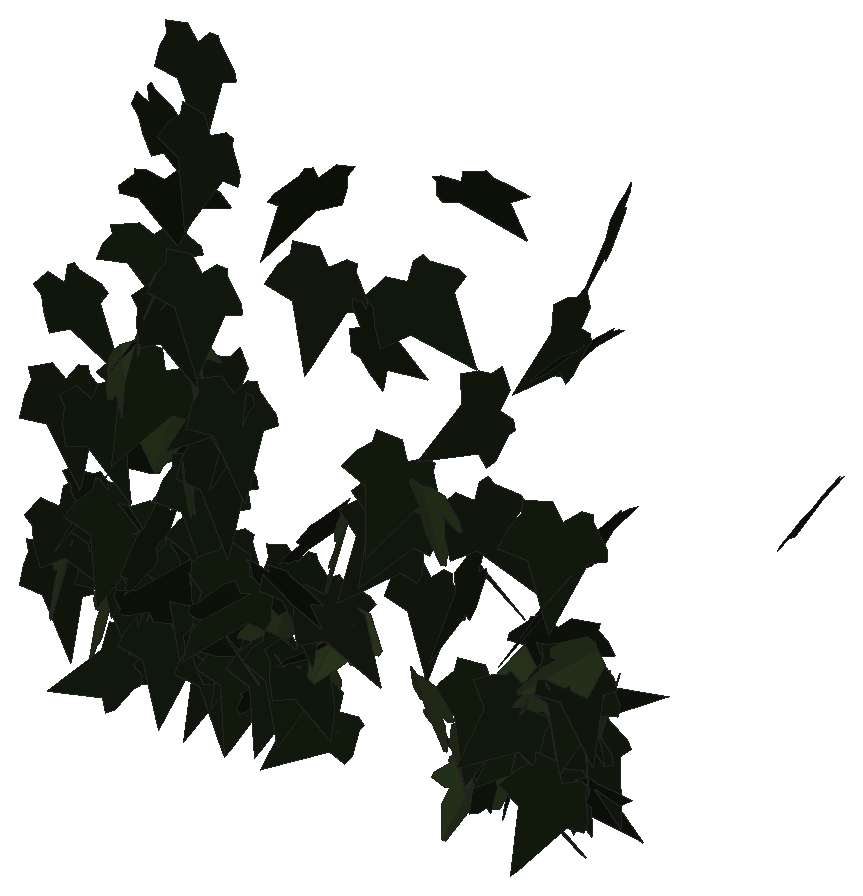
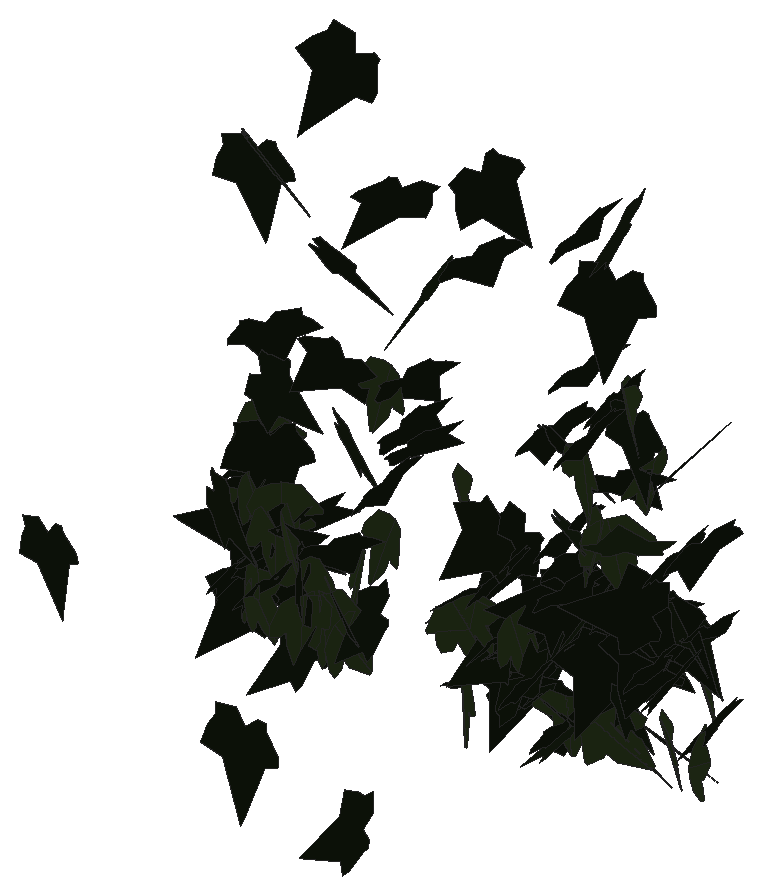
# SketchUp Ruby script. Lengths in inches.
U = 1.inch
M = Sketchup.active_model
def pt(a) = Geom::Point3d.new(a.map { |v| v * U })
def face(e, loops, mat)
  f = e.add_face(loops[0].map { |a| pt(a) })
  loops[1..].each { |l| e.add_face(l.map { |a| pt(a) }).erase! }
  f.material = f.back_material = mat if mat
  f
end
# faces: each face lists its corners as indices into pts; further lists are holes
def faces(e, pts, list, mat = nil) = list.each { |f| face(e, (f[0].is_a?(Array) ? f : [f]).map { |l| l.map { |i| pts[i] } }, mat) }
# xy, xz, yz: faces in a plane at the given z, y or x. An outline is a flat list of corners, or four numbers for a rectangle; further outlines are holes
def ring(l) = l.size == 4 ? [[l[0], l[1]], [l[2], l[1]], [l[2], l[3]], [l[0], l[3]]] : l.each_slice(2).to_a
def flat(e, list, mat, &to3) = list.each { |f| face(e, (f[0].is_a?(Array) ? f : [f]).map { |l| ring(l).map { |u, v| to3.(u, v) } }, mat) }
def xy(e, z, list, mat = nil) = flat(e, list, mat) { |x, y| [x, y, z] }
def xz(e, y, list, mat = nil) = flat(e, list, mat) { |x, z| [x, y, z] }
def yz(e, x, list, mat = nil) = flat(e, list, mat) { |y, z| [x, y, z] }
def lines(e, pts, list) = list.each { |a, b| e.add_line(pt(pts[a]), pt(pts[b])) }
# prism: a flat outline (further loops are holes) pulled along v
def prism(e, loops, v, mat = nil)
  f = face(e, loops, mat); d = Geom::Vector3d.new(v.map { |x| x * U })
  f.pushpull(f.normal.samedirection?(d) ? d.length : -d.length)
end
def box(e, o, s, mat = nil) = prism(e, [[o, [o[0] + s[0], o[1], o[2]], [o[0] + s[0], o[1] + s[1], o[2]], [o[0], o[1] + s[1], o[2]]]], [0, 0, s[2]], mat)
def at(x, y, z, deg = 0) = Geom::Transformation.translation(pt([x, y, z])) * Geom::Transformation.rotation(ORIGIN, Z_AXIS, deg.degrees)
def axes(o, x, y, z) = Geom::Transformation.new([*x, 0, *y, 0, *z, 0, *pt(o).to_a, 1])
def part(name) = M.definitions.add(name)
# library, detail: a bought-in or finely detailed component or shape, given as its bounding box
def library(name, o, s) = part(name).tap { |d| box(d.entities, o, s) }
def detail(e, o, s) = box(e.add_group.entities, o, s)
def put(e, d, t, mat = nil) = e.add_instance(d, t).tap { |i| i.material = mat if mat }
def group(e, t, mat = nil) = e.add_group.tap { |g| g.transformation = t; g.material = mat if mat }.entities
root = M.entities
M.materials.add("efeu1").color = [18, 25, 13]
M.materials.add("efeu2").color = [43, 57, 29]
c1 = part("ivyleaf_9")
p = [[1.54,2.16,1.25],[1.36,2.04,1.19],[-0.21,0.99,0.68],[-0.71,1.11,0.82],[-0.85,0.86,0.67],[-0.8,0.17,0.21],
  [-0.9,-0.01,0.1],[-0.67,-0.16,-0.02],[-0.08,-0.08,-0.05],[-0.03,-0.6,-0.4],[0.65,-0.88,-0.66],[0.83,-0.6,-0.49],
  [1.29,-0.42,-0.43],[1.8125,-0.07,-0.26],[1.21,0.44,0.15]]
faces(c1.entities,p,[[0,1,2,3,4,5,6,7,8,9,10,11,12,13,14]],"efeu1")
c2 = part("ivyleaf_10")
p = [[0,0.5,-0.03],[-0.0625,2.02,-0.43],[-0.19,2.01,-0.46],[-0.54,1.05,-0.29],[-0.52,0.625,-0.18],[-0.83,0.76,-0.28],
  [-1.16,0.64,-0.33],[-1.15,0.33,-0.24],[-0.77,-0.39,0.02],[-0.3,-0.51,0.16],[0.04,-0.48,0.23],[-0.02,2.01,-0.4375],
  [-0.06,2.01,-0.43],[0.04,-0.49,0.23],[0.67,-0.49,0.14],[1.38,0.36,-0.2],[1.375,0.51,-0.24],[0.81,0.65,-0.19],
  [0.62,0.59,-0.15],[0.6,1.09,-0.28],[0.5,1.23,-0.31]]
faces(c2.entities,p,[[0,1,2,3,4,5,6,7,8,9,10],[11,12,0,13,14,15,16,17,18,19,20]],"efeu2")
put(root,c1,axes([610.64,121.71,306.62],[1.08551,0.69081,0.17384],[-0.15041,-0.08744,1.28666],[0.69629,-1.09586,0.00692]))
put(root,c1,axes([614.42,122.42,308.86],[-1.10207,-0.62143,0.03852],[-0.02912,-0.02679,-1.26517],[0.62194,-1.10242,0.00903]))
put(root,c1,axes([618.05,122.52,322.72],[-0.41408,-1.25309,-0.00492],[0.02508,-0.00311,-1.3195],[1.25285,-0.4141,0.02479]))
put(root,c1,axes([610.88,121.58,309.32],[-0.86146,0.89959,0.31349],[-0.24442,0.19979,-1.24499],[-0.92076,-0.89469,0.03719]))
put(root,c1,axes([617.8,122.21,326.47],[-0.25735,0.84043,-0.97979],[0.18728,-0.9642,-0.87624],[-1.2772,-0.31073,0.06893]))
put(root,c1,axes([613.96,122.34,316.17],[0.01708,-1.28705,-0.21282],[0.02089,0.21308,-1.28695],[1.30436,0.01344,0.0234]))
put(root,c1,axes([621.48,122.69,315.9],[-0.56375,-1.14112,0.16814],[-0.04683,-0.16435,-1.27241],[1.15249,-0.56486,0.03055]))
put(root,c1,axes([621.02,122.91,312.99],[-0.6656,-0.96256,0.5463],[-0.13452,-0.5624,-1.15482],[1.09858,-0.65206,0.18958]))
put(root,c1,axes([626.11,122.16,319.94],[-1.26166,0.2257,0.22147],[-0.2124,0.07001,-1.28131],[-0.23426,-1.27904,-0.03105]))
put(root,c2,axes([623.17,121.78,307.72],[-1.10794,0.56302,-0.13169],[0.1236,-0.04743,-1.24271],[-0.56485,-1.11473,-0.01363]))
put(root,c1,axes([628.68,122.52,305.29],[-1.05697,-0.60589,-0.18367],[0.17173,0.06967,-1.21806],[0.60938,-1.07055,0.02468]))
put(root,c1,axes([612.33,122.9,326],[-0.13885,-1.22781,0.42385],[-0.04229,-0.42177,-1.23562],[1.29822,-0.14506,0.00508]))
put(root,c2,axes([606.21,122.37,307.05],[0.79546,-0.92167,0.22736],[0.14224,-0.17755,-1.21744],[0.93858,0.80804,-0.00818]))
put(root,c2,axes([629.6,122.72,310.77],[0.07849,0.50649,-1.15391],[-0.8251,-0.85322,-0.43063],[-0.9525,0.78083,0.27794]))
put(root,c1,axes([608.72,122.79,309.53],[-0.62675,-1.11366,-0.00561],[0.1299,-0.06671,-1.26955],[1.10607,-0.62321,0.14592]))
put(root,c1,axes([609.25,122.22,303.62],[-1.09457,0.48971,0.33079],[-0.38392,-0.05992,-1.18167],[-0.44927,-1.14189,0.20387]))
put(root,c1,axes([606.38,121.96,309.07],[0.53454,-1.03447,-0.68023],[-0.04926,0.72256,-1.13756],[1.23709,0.47576,0.24863]))
put(root,c1,axes([626.62,123.11,307.45],[-0.57289,-0.82169,0.75071],[-0.32175,-0.68601,-0.9964],[1.06546,-0.64897,0.10276]))
put(root,c1,axes([622.4375,121.84,323.98],[0.13632,-0.81519,-1.05838],[0.1734,1.06567,-0.79847],[1.32462,-0.05562,0.21344]))
put(root,c1,axes([616.21,121.72,309.96],[1.23253,0.18978,-0.27365],[-0.27289,-0.02575,-1.24695],[-0.19087,1.26228,0.0157]))
put(root,c1,axes([607.3,121.91,309.33],[-0.67909,1.04755,-0.01213],[0.00582,-0.01068,-1.24841],[-1.0476,-0.67911,0.00092]))
put(root,c1,axes([613.58,121.23,307.36],[0.30178,0.83143,-1.063],[0.10534,1.07142,0.86792],[1.34542,-0.27038,0.17048]))
put(root,c1,axes([625.12,121.62,329.21],[1.19782,0.60261,-0.08137],[-0.06909,-0.04373,-1.34084],[-0.60414,1.19978,-0.008]))
put(root,c1,axes([628.69,122.7,315.92],[-0.59992,-1.12921,-0.35348],[0.12369,0.3343,-1.27785],[1.17676,-0.61082,-0.0459]))
put(root,c2,axes([624.63,121.76,305.61],[-0.75004,0.83417,0.54696],[-0.40946,0.36656,-1.12051],[-0.90959,-0.85286,0.05339]))
put(root,c1,axes([628.76,122.77,313.43],[-0.79843,0.57207,-0.85057],[0.41945,-0.80142,-0.93275],[-0.93531,-0.84776,0.3078]))
put(root,c2,axes([608.98,122.27,315.89],[-0.0518,1.24886,-0.16149],[0.00177,-0.16155,-1.24993],[-1.25926,-0.0516,0.00489]))
put(root,c2,axes([622.96,122.24,315.18],[-1.21093,0.34721,-0.14431],[0.10606,-0.15147,-1.25441],[-0.36074,-1.21006,0.11562]))
put(root,c2,axes([610.1,122.39,318.86],[0.61528,-1.10104,-0.14151],[-0.05967,0.12876,-1.26125],[1.10849,0.61807,0.01065]))
put(root,c1,axes([610.26,122.25,326.84],[0.97872,-0.90264,-0.37513],[-0.27172,0.2587,-1.3314],[0.93897,1.01572,0.00573]))
put(root,c1,axes([621.17,123.27,313.94],[-0.43563,-1.10953,0.50024],[-0.19344,-0.46145,-1.19194],[1.20162,-0.47653,-0.01053]))
put(root,c1,axes([610.03,123.12,315.4375],[-0.94207,-0.86611,-0.0184],[0.10671,-0.08904,-1.27227],[0.8597,-0.93804,0.13776]))
put(root,c1,axes([611.83,123.1,320.05],[-0.12253,-1.29694,0.07763],[0.10807,-0.08788,-1.29757],[1.29475,-0.1154,0.11566]))
put(root,c1,axes([615.54,123.15,305.48],[-0.37744,-1.16583,0.13824],[-0.05775,-0.1266,-1.2253],[1.17258,-0.38151,-0.01585]))
put(root,c1,axes([605.84,122.84,313.69],[0.06407,-1.26811,-0.30251],[-0.05005,0.30026,-1.26928],[1.30273,0.0739,-0.03389]))
put(root,c1,axes([615.89,123.31,305.58],[-0.17694,-1.16768,0.36339],[0.12049,-0.38204,-1.16892],[1.21697,-0.13195,0.16857]))
put(root,c1,axes([606.15,122.52,317.94],[0.66299,-1.04852,-0.38198],[0.00986,0.44979,-1.21756],[1.11589,0.619,0.2377]))
put(root,c1,axes([610.53,122.57,318.89],[0.49322,-1.06588,-0.48193],[-0.1739,0.45039,-1.17411],[1.15677,0.52217,0.02897]))
put(root,c1,axes([624.61,122.88,312.42],[-1.05158,0.42026,-0.5931],[0.54593,-0.23207,-1.13239],[-0.47994,-1.18479,0.01143]))
put(root,c1,axes([624.92,122.55,315.55],[-0.18193,-0.48036,-1.18869],[0.90048,0.80674,-0.46383],[0.91261,-0.89177,0.22069]))
put(root,c1,axes([629.34,122.79,324.14],[-1.21164,0.48754,-0.13641],[0.11685,-0.07495,-1.30579],[-0.49259,-1.21699,0.02578]))
put(root,c1,axes([610.33,123.26,304.92],[-0.22196,-1.22239,0.01612],[-0.00173,-0.01607,-1.24238],[1.2225,-0.22196,0.00117]))
put(root,c1,axes([610,122.08,317.65],[-0.33468,1.20466,0.20124],[-0.03174,0.20001,-1.25008],[-1.22094,-0.33542,-0.02267]))
put(root,c1,axes([607.89,122.68,309.62],[0.26067,0.23996,-1.31938],[-1.10691,-0.72024,-0.34969],[-0.75702,1.13576,0.057]))
put(root,c1,axes([612.57,123.53,309.52],[-0.42148,-1.18848,0.26343],[0.03035,-0.28894,-1.25504],[1.21695,-0.40441,0.12253]))
put(root,c1,axes([622.12,123.35,311.06],[0.05059,-1.26886,0.1505],[-0.01329,-0.15114,-1.26973],[1.27769,0.04867,-0.01916]))
put(root,c1,axes([613.57,122.9375,316.04],[-1.25572,0.27052,0.00943],[-0.00813,0.00705,-1.28452],[-0.27056,-1.25573,-0.00518]))
put(root,c1,axes([608.35,123.09,307.53],[-0.71403,-0.64221,-0.79349],[0.71476,0.37683,-0.94817],[0.72883,-0.99873,0.15248]))
put(root,c1,axes([628.94,123.18,310.16],[0.20312,-1.26985,-0.15202],[-0.01385,0.15174,-1.28595],[1.27884,0.20334,0.01022]))
put(root,c2,axes([618.35,123.02,312.01],[0.68633,-1.06488,0.05864],[0.03169,-0.04933,-1.26689],[1.06602,0.68706,-0.00009]))
put(root,c1,axes([610.78,122.4,323.9],[0.87505,0.89133,-0.58902],[-0.41747,-0.41558,-1.24906],[-0.98343,0.96951,0.00612]))
put(root,c1,axes([617.4,123.81,303.8],[-0.91132,-0.67348,0.51749],[-0.14345,-0.62605,-1.0674],[0.83713,-0.84045,0.38043]))
put(root,c2,axes([611.78,122.5,312.37],[-0.53194,1.07296,0.40355],[-0.33055,0.28241,-1.1866],[-1.09765,-0.60502,0.16177]))
put(root,c1,axes([619.92,122.3,321.125],[0.94121,-0.29583,-0.85126],[-0.59296,0.72361,-0.90709],[0.67864,1.04255,0.38804]))
put(root,c1,axes([604.95,123.47,305.77],[0.26106,-1.24339,0.04769],[0.0008,-0.04856,-1.27046],[1.2443,0.2609,-0.00919]))
put(root,c1,axes([611.16,123.72,307.77],[-0.19868,-1.24298,0.18906],[-0.00544,-0.19056,-1.25852],[1.25726,-0.19725,0.02443]))
put(root,c1,axes([606.84,123.17,313.07],[0.46466,-1.16887,-0.33838],[-0.06248,0.33882,-1.25617],[1.21526,0.46434,0.0648]))
put(root,c1,axes([624.64,123.7,307.37],[-0.62265,-1.11776,-0.06517],[0.163,-0.01672,-1.27063],[1.10773,-0.62583,0.15034]))
put(root,c1,axes([629.53,122.44,323.48],[-0.01836,1.30968,-0.03439],[-0.21941,-0.03698,-1.29123],[-1.29163,-0.01234,0.21983]))
put(root,c1,axes([628.72,123.73,309.28],[-0.44236,-1.16717,0.01331],[0.12888,-0.06299,-1.23999],[1.16011,-0.43805,0.14283]))
put(root,c1,axes([613.59,122.82,305.74],[1.18002,-0.45086,-0.2997],[-0.26987,0.1332,-1.26292],[0.46933,1.21017,0.02735]))
put(root,c2,axes([623.77,123.85,303.54],[-0.22456,-1.00494,0.74621],[0.11775,-0.77172,-1.00386],[1.24614,-0.10818,0.22933]))
put(root,c1,axes([628.08,123.58,309.57],[0.71181,-1.1333,0.21021],[0.1288,-0.16731,-1.33816],[1.14542,0.7231,0.01984]))
put(root,c1,axes([611.6875,123.68,311.5625],[-0.1668,-1.26165,-0.18275],[-0.00219,0.18459,-1.27236],[1.27482,-0.16476,-0.0261]))
put(root,c1,axes([612.17,123.73,312.55],[0.14964,-1.27223,-0.00027],[-0.00779,-0.00065,-1.28098],[1.27221,0.14964,-0.00781]))
put(root,c1,axes([613.82,123.74,304.82],[-0.98697,-0.64082,-0.43417],[0.4223,0.14384,-1.17228],[0.64871,-1.06861,0.10257]))
put(root,c1,axes([627.19,123.96,306.92],[-1.11125,-0.55593,0.28897],[-0.255,-0.13614,-1.24253],[0.57231,-1.14011,0.00747]))
put(root,c1,axes([615.73,123.79,309.24],[0.255,-1.25601,0.00718],[0.00007,-0.00731,-1.28163],[1.25603,0.255,-0.00138]))
put(root,c1,axes([608.42,122.6875,307.99],[0.93993,0.85284,-0.09548],[-0.06415,-0.07138,-1.26914],[-0.85577,0.94207,-0.00973]))
put(root,c1,axes([616.06,123.4,305.9],[0.47227,-1.11192,-0.44039],[-0.09122,0.43862,-1.20526],[1.19247,0.47392,0.08222]))
put(root,c2,axes([614.92,123.71,306.91],[-0.13621,-1.20094,0.332],[0.10479,-0.34384,-1.20076],[1.24157,-0.10273,0.13776]))
put(root,c1,axes([607.33,124.07,308.14],[-0.08153,-1.26472,0.13322],[0.01535,-0.13446,-1.26712],[1.27162,-0.07946,0.02383]))
put(root,c1,axes([607.84,123.84,307.58],[0.49611,-1.15033,0.0306],[0.01031,-0.02888,-1.25275],[1.15069,0.49622,-0.00196]))
put(root,c1,axes([625.79,124.17,305.99],[-0.27718,-0.01712,-1.20854],[1.06176,-0.5959,-0.23507],[-0.57752,-1.08733,0.14786]))
put(root,c2,axes([607.08,123.625,304.83],[0.80979,-0.96446,-0.08158],[-0.05467,0.06063,-1.25934],[0.96636,0.81162,-0.00288]))
put(root,c1,axes([610.21,123.51,304.02],[-1.08028,0.51894,0.31171],[-0.29999,0.09493,-1.19769],[-0.52581,-1.12034,0.0429]))
put(root,c1,axes([625.23,123.0625,304.6],[-0.5285,0.07431,-1.11335],[-1.11096,0.07989,0.5327],[0.1041,1.22983,0.03267]))
put(root,c1,axes([615.25,122.84,304.55],[0.5785,1.10722,0.09654],[0.03975,0.08815,-1.24923],[-1.11071,0.57984,0.00557]))
put(root,c1,axes([606.4375,123.99,307.73],[0.43125,-1.19203,-0.13145],[-0.01514,0.13427,-1.26726],[1.19916,0.43038,0.03128]))
put(root,c1,axes([627.93,123.41,311.11],[0.62878,0.88608,-0.70008],[-0.3885,-0.58264,-1.08637],[-1.06034,0.73892,-0.0171]))
put(root,c1,axes([611.13,123.39,309.03],[0.85249,-0.69042,-0.61294],[-0.33422,0.54691,-1.08088],[0.86062,0.89628,0.1874]))
put(root,c1,axes([609.21,124.02,306.22],[-0.82615,0.55261,-0.75821],[0.64475,-0.39953,-0.99372],[-0.68159,-1.04775,-0.02098]))
put(root,c1,axes([612.11,124,312.89],[-1.16656,0.47717,-0.12141],[0.03965,-0.22015,-1.2463],[-0.49078,-1.15201,0.18788]))
put(root,c2,axes([609.81,123.92,313.21],[-0.86619,-0.87222,0.29976],[-0.22689,-0.19707,-1.22906],[0.89394,-0.89516,-0.0215]))
put(root,c1,axes([613.99,124.47,304.65],[1.18535,-0.48028,-0.56029],[0.54687,-0.14012,1.27708],[-0.4955,-1.30358,0.06916]))
put(root,c1,axes([622.12,123.69,304.99],[1.16458,-0.49667,-0.09502],[-0.08504,0.04282,-1.26605],[0.49848,1.16766,0.00601]))
put(root,c1,axes([611.84,124.49,304.27],[-1.06825,-0.32178,-0.57465],[0.62448,-0.14693,-1.07859],[0.20928,-1.20407,0.2852]))
put(root,c2,axes([626.86,124.14,309.08],[-1.00867,-0.76342,0.01216],[0.23802,-0.33355,-1.19686],[0.72547,-0.952,0.40959]))
put(root,c1,axes([615.7,122.9,305.39],[0.7365,0.63723,0.79432],[0.30162,0.79981,-0.92129],[-0.97264,0.73054,0.31578]))
put(root,c1,axes([616.85,124.01,308.22],[0.40291,-1.12234,-0.44563],[0.27027,0.54167,-1.11988],[1.17694,0.25983,0.40972]))
put(root,c1,axes([627.71,124.46,306.28],[-0.07646,-1.24239,-0.11518],[0.05052,0.11222,-1.24398],[1.24669,-0.08074,0.04335]))
put(root,c1,axes([625.74,124.18,305.27],[0.36803,0.018,-1.29043],[1.26842,0.24243,0.36514],[0.23801,-1.31981,0.04947]))
put(root,c2,axes([611.34,123.98,316.17],[-1.13677,0.53844,0.18506],[-0.32828,-0.28222,-1.1954],[-0.46518,-1.11662,0.39136]))
put(root,c1,axes([611.72,124.51,303.97],[-0.03799,-1.25343,-0.06295],[-0.00193,0.06304,-1.254],[1.25501,-0.03785,-0.00384]))
put(root,c2,axes([624.76,124.01,304.65],[-0.99521,-0.76625,0.11351],[-0.07413,-0.08974,-1.25576],[0.77106,-0.99763,0.02578]))
put(root,c2,axes([610.34,124.17,313.3],[-0.73977,0.91598,-0.45565],[0.2518,-0.38198,-1.17668],[-0.99158,-0.78036,0.04114]))
put(root,c2,axes([617.34,124.32,306.86],[-0.91224,-0.42045,0.7532],[-0.6267,-0.43024,-0.9992],[0.59274,-1.10199,0.10274]))
put(root,c2,axes([611.77,124.15,304.64],[1.21201,0.29471,0.06526],[0.05148,0.06428,-1.24631],[-0.29743,1.21206,0.05023]))
put(root,c2,axes([628.08,124.39,309.25],[0.08324,-1.24369,0.17658],[-0.00032,-0.17699,-1.24641],[1.25616,0.08237,-0.01202]))
put(root,c2,axes([627.13,124.14,308.06],[-0.49352,-1.16352,-0.08017],[0.05147,0.06523,-1.26367],[1.16515,-0.49571,0.02187]))
put(root,c2,axes([625.86,123.96,305.98],[1.20803,-0.07189,-0.3706],[-0.32991,0.40288,-1.15356],[0.18349,1.19765,0.3658]))
put(root,c2,axes([604.52,124.9375,304.66],[0.21695,-0.40986,1.14936],[0.70558,-0.91031,-0.45779],[0.99558,0.73446,0.07398]))
put(root,c1,axes([613.23,124.65,305.63],[0.04297,-1.24795,-0.07814],[-0.01623,0.07763,-1.24862],[1.25029,0.04389,-0.01352]))
put(root,c2,axes([617.25,124.39,307.28],[0.92224,0.70496,-0.47769],[-0.43205,-0.21943,-1.15795],[-0.73382,1.01516,0.08143]))
put(root,c2,axes([626.25,124.42,308.09],[0.55464,-1.12895,0.04152],[0.02735,-0.03283,-1.2578],[1.12939,0.55522,0.01007]))
put(root,c2,axes([609.41,124.64,304.58],[0.69308,0.56764,-0.87375],[-0.86186,-0.2774,-0.86386],[-0.58554,1.08021,0.2373]))
put(root,c1,axes([616.34,123.33,310.66],[0.45934,0.78995,0.89487],[0.26645,0.86679,-0.90193],[-1.16354,0.51034,0.14673]))
put(root,c1,axes([609.96,123.84,307.46],[0.79806,0.9655,-0.09491],[-0.07691,-0.05955,-1.25245],[-0.9671,0.80147,0.02128]))
put(root,c2,axes([629.17,124.85,308.25],[0.41248,-1.15487,0.20059],[0.09235,-0.17997,-1.22604],[1.16851,0.42189,0.02609]))
put(root,c1,axes([626.81,124.86,305.53],[0.31625,-1.14285,-0.3785],[-0.01396,0.38784,-1.1827],[1.20382,0.30473,0.08572]))
put(root,c2,axes([625.24,124.72,304.5625],[-0.72216,-1.01441,-0.07105],[0.11881,0.00239,-1.24156],[1.00993,-0.72564,0.09525]))
put(root,c1,axes([611.125,124.72,304.01],[0.76084,-0.96644,-0.22548],[0.08747,0.34832,-1.19781],[0.98853,0.71301,0.27953]))
put(root,c1,axes([628.13,124.23,304.2],[1.14899,0.41498,0.05925],[0.05753,0.01512,-1.22162],[-0.41522,1.15042,-0.00532]))
put(root,c2,axes([616.78,124.66,304.07],[0.85791,-0.86703,-0.27942],[0.01675,0.39878,-1.18597],[0.91079,0.80936,0.285]))
put(root,c2,axes([627.17,125.3,305],[0.23534,-1.16667,0.30849],[0.01937,-0.3106,-1.18946],[1.20661,0.23254,-0.04108]))
put(root,c1,axes([627.99,125.25,306.13],[0.34284,-1.15534,-0.25454],[-0.0063,0.26323,-1.20325],[1.18303,0.33622,0.06735]))
put(root,c1,axes([627.49,124.51,307.45],[0.61607,-0.00289,1.09485],[1.08199,0.19367,-0.60832],[-0.16738,1.24126,0.09746]))
put(root,c2,axes([627.76,124.99,305.98],[0.91291,-0.8154,-0.0325],[0.24154,0.31658,-1.15792],[0.77948,0.85688,0.39687]))
put(root,c1,axes([624.97,124.88,303.09],[1.17931,-0.37647,-0.00417],[0.00408,0.02649,-1.23766],[0.37647,1.17902,0.02648]))
put(root,c1,axes([607.3125,124.58,310.63],[0.7151,-0.01452,1.03007],[0.98671,0.37006,-0.67978],[-0.2961,1.19811,0.22245]))
put(root,c1,axes([604.77,129.18,316.56],[-0.31679,-1.24108,-0.02155],[0.88547,-0.21036,-0.90155],[0.86988,-0.23784,0.90986]))
put(root,c1,axes([604.65,131.88,323.15],[0.13834,-1.28946,0.08847],[0.02102,-0.08672,-1.29681],[1.29232,0.13944,0.01162]))
put(root,c1,axes([629.79,135.62,311.3],[-0.34934,1.18854,0.11043],[-0.01569,0.11048,-1.23871],[-1.19355,-0.34932,-0.01604]))
put(root,c1,axes([612.89,136.39,303.82],[1.11261,-0.5802,0.29384],[0.24788,-0.16001,-1.25452],[0.60128,1.13958,-0.02655]))
put(root,c1,axes([619.25,135.98,306.05],[-0.06066,1.38934,0.22926],[-0.00975,0.22905,-1.39066],[-1.40809,-0.06144,-0.00025]))
put(root,c1,axes([618.8,138.375,318.29],[-0.9484,0.61045,-0.79131],[0.67583,-0.41192,-1.12777],[-0.73625,-1.16446,-0.01589]))
